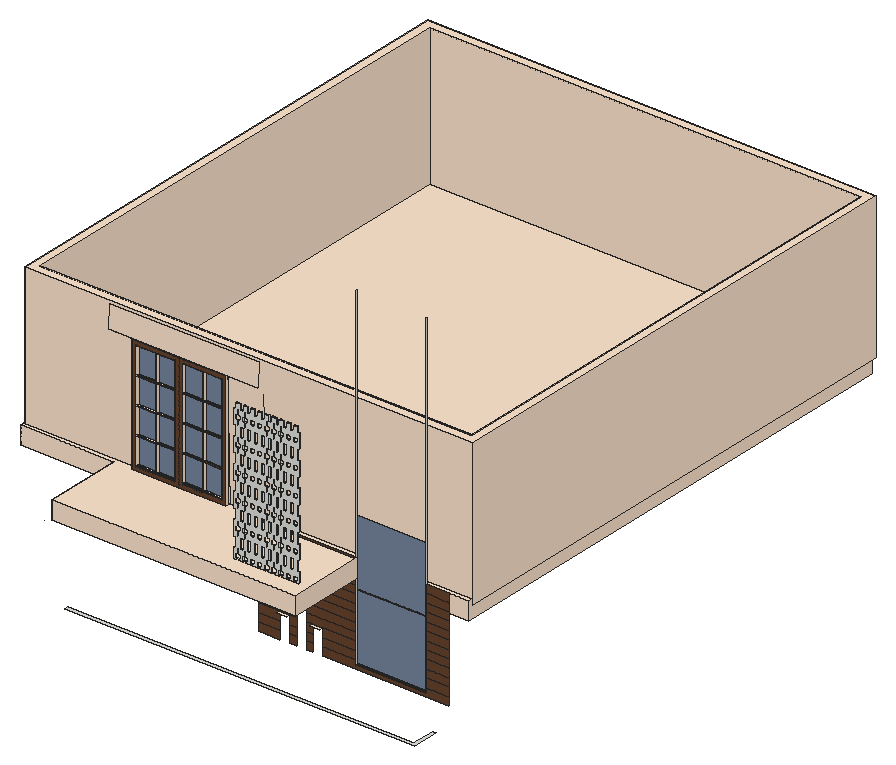
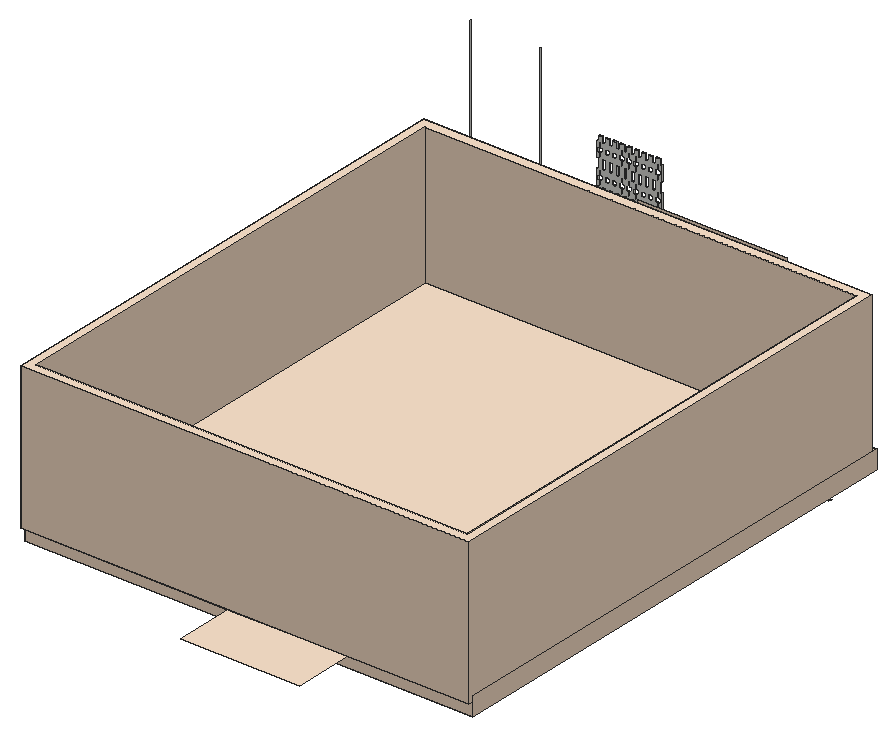
# SketchUp Ruby script. Lengths in inches.
U = 1.inch
M = Sketchup.active_model
def pt(a) = Geom::Point3d.new(a.map { |v| v * U })
def face(e, loops, mat)
  f = e.add_face(loops[0].map { |a| pt(a) })
  loops[1..].each { |l| e.add_face(l.map { |a| pt(a) }).erase! }
  f.material = f.back_material = mat if mat
  f
end
# faces: each face lists its corners as indices into pts; further lists are holes
def faces(e, pts, list, mat = nil) = list.each { |f| face(e, (f[0].is_a?(Array) ? f : [f]).map { |l| l.map { |i| pts[i] } }, mat) }
# xy, xz, yz: faces in a plane at the given z, y or x. An outline is a flat list of corners, or four numbers for a rectangle; further outlines are holes
def ring(l) = l.size == 4 ? [[l[0], l[1]], [l[2], l[1]], [l[2], l[3]], [l[0], l[3]]] : l.each_slice(2).to_a
def flat(e, list, mat, &to3) = list.each { |f| face(e, (f[0].is_a?(Array) ? f : [f]).map { |l| ring(l).map { |u, v| to3.(u, v) } }, mat) }
def xy(e, z, list, mat = nil) = flat(e, list, mat) { |x, y| [x, y, z] }
def xz(e, y, list, mat = nil) = flat(e, list, mat) { |x, z| [x, y, z] }
def yz(e, x, list, mat = nil) = flat(e, list, mat) { |y, z| [x, y, z] }
def lines(e, pts, list) = list.each { |a, b| e.add_line(pt(pts[a]), pt(pts[b])) }
# prism: a flat outline (further loops are holes) pulled along v
def prism(e, loops, v, mat = nil)
  f = face(e, loops, mat); d = Geom::Vector3d.new(v.map { |x| x * U })
  f.pushpull(f.normal.samedirection?(d) ? d.length : -d.length)
end
def box(e, o, s, mat = nil) = prism(e, [[o, [o[0] + s[0], o[1], o[2]], [o[0] + s[0], o[1] + s[1], o[2]], [o[0], o[1] + s[1], o[2]]]], [0, 0, s[2]], mat)
def at(x, y, z, deg = 0) = Geom::Transformation.translation(pt([x, y, z])) * Geom::Transformation.rotation(ORIGIN, Z_AXIS, deg.degrees)
def axes(o, x, y, z) = Geom::Transformation.new([*x, 0, *y, 0, *z, 0, *pt(o).to_a, 1])
def part(name) = M.definitions.add(name)
# library, detail: a bought-in or finely detailed component or shape, given as its bounding box
def library(name, o, s) = part(name).tap { |d| box(d.entities, o, s) }
def detail(e, o, s) = box(e.add_group.entities, o, s)
def put(e, d, t, mat = nil) = e.add_instance(d, t).tap { |i| i.material = mat if mat }
def group(e, t, mat = nil) = e.add_group.tap { |g| g.transformation = t; g.material = mat if mat }.entities
root = M.entities
M.materials.add("C01_Vanilla_Cream").color = [255, 230, 206]
M.materials.add("Glass_Mirror_01").color = [119, 135, 160]
M.materials.add("Wood_Veneer_15_1K").color = [103, 69, 45]
xy(root,193.67,[[105.48,138.27,465.23,138.27,465.23,165.41,462.4,165.41,462.4,141.07,105.48,141.07]])
xy(root,203.87,[[357,198,429,199.5]])
xy(root,225.8,[[278.18,194.51,288.54,198],[312.12,194.51,322.48,198]],"C01_Vanilla_Cream")
xy(root,243.16,[[296.18,194.51,306.54,198]],"C01_Vanilla_Cream")
xy(root,292.23,[[282.27,137.21,285.76,138.74],[289.68,137.21,293.17,138.74],[297.09,137.21,300.58,138.74],[304.5,137.21,307.99,138.74],[311.91,137.21,315.4,138.74],
  [319.32,137.21,322.81,138.74],[326.73,137.21,330.22,138.74],[334.14,137.21,337.63,138.74],[341.55,137.21,345.04,138.74]])
xz(root,137.21,[[[282.27,292.23,285.76,292.23,285.76,297.49,289.68,297.49,289.68,292.23,293.17,292.23,293.17,297.49,297.09,297.49,297.09,292.23,300.58,292.23,300.58,297.49,304.5,297.49,304.5,292.23,307.99,292.23,307.99,297.49,311.91,297.49,311.91,292.23,315.4,292.23,315.4,297.49,319.32,297.49,319.32,292.23,322.81,292.23,322.81,297.49,326.73,297.49,326.73,292.23,330.22,292.23,330.22,297.49,334.14,297.49,334.14,292.23,337.63,292.23,337.63,297.49,341.55,297.49,341.55,292.23,345.04,292.23,345.04,297.49,347,297.49,347,312.59,345.04,312.59,345.04,323.12,347,323.12,347,338.22,345.04,338.22,345.04,348.75,347,348.75,347,363.84,345.04,363.84,345.04,374.38,347,374.38,347,389.47,345.04,389.47,345.04,400.01,347,400.01,347,415.1,345.04,415.1,345.04,425.64,347,425.64,347,440.73,345.04,440.73,345.04,446,341.55,446,341.55,440.73,337.63,440.73,337.63,446,334.14,446,334.14,440.73,330.22,440.73,330.22,446,326.73,446,326.73,440.73,322.81,440.73,322.81,446,319.32,446,319.32,440.73,315.4,440.73,315.4,446,311.91,446,311.91,440.73,307.99,440.73,307.99,446,304.5,446,304.5,440.73,300.58,440.73,300.58,446,297.09,446,297.09,440.73,293.17,440.73,293.17,446,289.68,446,289.68,440.73,285.76,440.73,285.76,446,282.27,446,282.27,440.73,280.31,440.73,280.31,425.64,282.27,425.64,282.27,415.1,280.31,415.1,280.31,400.01,282.27,400.01,282.27,389.47,280.31,389.47,280.31,374.38,282.27,374.38,282.27,363.84,280.31,363.84,280.31,348.75,282.27,348.75,282.27,338.22,280.31,338.22,280.31,323.12,282.27,323.12,282.27,312.59,280.31,312.59,280.31,297.49,282.27,297.49],[312.78,297.09,312.78,302.36,310.82,302.36,310.82,307.72,312.78,307.72,312.78,312.99,314.53,312.99,314.53,307.72,316.49,307.72,316.49,302.36,314.53,302.36,314.53,297.09],[305.37,297.09,305.37,302.36,303.41,302.36,303.41,307.72,305.37,307.72,305.37,312.99,307.12,312.99,307.12,307.72,309.08,307.72,309.08,302.36,307.12,302.36,307.12,297.09],[312.78,399.61,312.78,404.88,310.82,404.88,310.82,410.24,312.78,410.24,312.78,415.5,314.53,415.5,314.53,410.24,316.49,410.24,316.49,404.88,314.53,404.88,314.53,399.61],[312.78,373.98,312.78,379.25,310.82,379.25,310.82,384.61,312.78,384.61,312.78,389.875,314.53,389.875,314.53,384.61,316.49,384.61,316.49,379.25,314.53,379.25,314.53,373.98],[312.78,425.24,312.78,430.51,310.82,430.51,310.82,435.86,312.78,435.86,312.78,441.13,314.53,441.13,314.53,435.86,316.49,435.86,316.49,430.51,314.53,430.51,314.53,425.24],[312.78,322.72,312.78,327.99,310.82,327.99,310.82,333.35,312.78,333.35,312.78,338.62,314.53,338.62,314.53,333.35,316.49,333.35,316.49,327.99,314.53,327.99,314.53,322.72],[305.37,399.61,305.37,404.88,303.41,404.88,303.41,410.24,305.37,410.24,305.37,415.5,307.12,415.5,307.12,410.24,309.08,410.24,309.08,404.88,307.12,404.88,307.12,399.61],[305.37,373.98,305.37,379.25,303.41,379.25,303.41,384.61,305.37,384.61,305.37,389.875,307.12,389.875,307.12,384.61,309.08,384.61,309.08,379.25,307.12,379.25,307.12,373.98],[305.37,425.24,305.37,430.51,303.41,430.51,303.41,435.86,305.37,435.86,305.37,441.13,307.12,441.13,307.12,435.86,309.08,435.86,309.08,430.51,307.12,430.51,307.12,425.24],[305.37,322.72,305.37,327.99,303.41,327.99,303.41,333.35,305.37,333.35,305.37,338.62,307.12,338.62,307.12,333.35,309.08,333.35,309.08,327.99,307.12,327.99,307.12,322.72],[312.78,348.35,312.78,353.62,310.82,353.62,310.82,358.98,312.78,358.98,312.78,364.24,314.53,364.24,314.53,358.98,316.49,358.98,316.49,353.62,314.53,353.62,314.53,348.35],[305.37,348.35,305.37,353.62,303.41,353.62,303.41,358.98,305.37,358.98,305.37,364.24,307.12,364.24,307.12,358.98,309.08,358.98,309.08,353.62,307.12,353.62,307.12,348.35],[342.42,297.09,342.42,302.36,340.46,302.36,340.46,307.72,342.42,307.72,342.42,312.99,344.17,312.99,344.17,307.72,346.13,307.72,346.13,302.36,344.17,302.36,344.17,297.09],[342.42,399.61,342.42,404.88,340.46,404.88,340.46,410.24,342.42,410.24,342.42,415.5,344.17,415.5,344.17,410.24,346.13,410.24,346.13,404.88,344.17,404.88,344.17,399.61],[342.42,425.24,342.42,430.51,340.46,430.51,340.46,435.86,342.42,435.86,342.42,441.13,344.17,441.13,344.17,435.86,346.13,435.86,346.13,430.51,344.17,430.51,344.17,425.24],[342.42,373.98,342.42,379.25,340.46,379.25,340.46,384.61,342.42,384.61,342.42,389.875,344.17,389.875,344.17,384.61,346.13,384.61,346.13,379.25,344.17,379.25,344.17,373.98],[342.42,322.72,342.42,327.99,340.46,327.99,340.46,333.35,342.42,333.35,342.42,338.62,344.17,338.62,344.17,333.35,346.13,333.35,346.13,327.99,344.17,327.99,344.17,322.72],[290.55,297.09,290.55,302.36,288.59,302.36,288.59,307.72,290.55,307.72,290.55,312.99,292.3,312.99,292.3,307.72,294.26,307.72,294.26,302.36,292.3,302.36,292.3,297.09],[290.55,399.61,290.55,404.88,288.59,404.88,288.59,410.24,290.55,410.24,290.55,415.5,292.3,415.5,292.3,410.24,294.26,410.24,294.26,404.88,292.3,404.88,292.3,399.61],[290.55,373.98,290.55,379.25,288.59,379.25,288.59,384.61,290.55,384.61,290.55,389.875,292.3,389.875,292.3,384.61,294.26,384.61,294.26,379.25,292.3,379.25,292.3,373.98],[290.55,425.24,290.55,430.51,288.59,430.51,288.59,435.86,290.55,435.86,290.55,441.13,292.3,441.13,292.3,435.86,294.26,435.86,294.26,430.51,292.3,430.51,292.3,425.24],[342.42,348.35,342.42,353.62,340.46,353.62,340.46,358.98,342.42,358.98,342.42,364.24,344.17,364.24,344.17,358.98,346.13,358.98,346.13,353.62,344.17,353.62,344.17,348.35],[290.55,322.72,290.55,327.99,288.59,327.99,288.59,333.35,290.55,333.35,290.55,338.62,292.3,338.62,292.3,333.35,294.26,333.35,294.26,327.99,292.3,327.99,292.3,322.72],[290.55,348.35,290.55,353.62,288.59,353.62,288.59,358.98,290.55,358.98,290.55,364.24,292.3,364.24,292.3,358.98,294.26,358.98,294.26,353.62,292.3,353.62,292.3,348.35],[335.01,297.09,335.01,302.36,333.05,302.36,333.05,307.72,335.01,307.72,335.01,312.99,336.76,312.99,336.76,307.72,338.72,307.72,338.72,302.36,336.76,302.36,336.76,297.09],[335.01,425.24,335.01,430.51,333.05,430.51,333.05,435.86,335.01,435.86,335.01,441.13,336.76,441.13,336.76,435.86,338.72,435.86,338.72,430.51,336.76,430.51,336.76,425.24],[327.6,297.09,327.6,302.36,325.64,302.36,325.64,307.72,327.6,307.72,327.6,312.99,329.35,312.99,329.35,307.72,331.31,307.72,331.31,302.36,329.35,302.36,329.35,297.09],[335.01,399.61,335.01,404.88,333.05,404.88,333.05,410.24,335.01,410.24,335.01,415.5,336.76,415.5,336.76,410.24,338.72,410.24,338.72,404.88,336.76,404.88,336.76,399.61],[335.01,373.98,335.01,379.25,333.05,379.25,333.05,384.61,335.01,384.61,335.01,389.875,336.76,389.875,336.76,384.61,338.72,384.61,338.72,379.25,336.76,379.25,336.76,373.98],[335.01,322.72,335.01,327.99,333.05,327.99,333.05,333.35,335.01,333.35,335.01,338.62,336.76,338.62,336.76,333.35,338.72,333.35,338.72,327.99,336.76,327.99,336.76,322.72],[327.6,373.98,327.6,379.25,325.64,379.25,325.64,384.61,327.6,384.61,327.6,389.875,329.35,389.875,329.35,384.61,331.31,384.61,331.31,379.25,329.35,379.25,329.35,373.98],[327.6,399.61,327.6,404.88,325.64,404.88,325.64,410.24,327.6,410.24,327.6,415.5,329.35,415.5,329.35,410.24,331.31,410.24,331.31,404.88,329.35,404.88,329.35,399.61],[327.6,425.24,327.6,430.51,325.64,430.51,325.64,435.86,327.6,435.86,327.6,441.13,329.35,441.13,329.35,435.86,331.31,435.86,331.31,430.51,329.35,430.51,329.35,425.24],[327.6,322.72,327.6,327.99,325.64,327.99,325.64,333.35,327.6,333.35,327.6,338.62,329.35,338.62,329.35,333.35,331.31,333.35,331.31,327.99,329.35,327.99,329.35,322.72],[283.14,297.09,283.14,302.36,281.18,302.36,281.18,307.72,283.14,307.72,283.14,312.99,284.89,312.99,284.89,307.72,286.85,307.72,286.85,302.36,284.89,302.36,284.89,297.09],[335.01,348.35,335.01,353.62,333.05,353.62,333.05,358.98,335.01,358.98,335.01,364.24,336.76,364.24,336.76,358.98,338.72,358.98,338.72,353.62,336.76,353.62,336.76,348.35],[283.14,399.61,283.14,404.88,281.18,404.88,281.18,410.24,283.14,410.24,283.14,415.5,284.89,415.5,284.89,410.24,286.85,410.24,286.85,404.88,284.89,404.88,284.89,399.61],[320.1875,297.09,320.1875,302.36,318.23,302.36,318.23,307.72,320.1875,307.72,320.1875,312.99,321.94,312.99,321.94,307.72,323.9,307.72,323.9,302.36,321.94,302.36,321.94,297.09],[283.14,373.98,283.14,379.25,281.18,379.25,281.18,384.61,283.14,384.61,283.14,389.875,284.89,389.875,284.89,384.61,286.85,384.61,286.85,379.25,284.89,379.25,284.89,373.98],[283.14,425.24,283.14,430.51,281.18,430.51,281.18,435.86,283.14,435.86,283.14,441.13,284.89,441.13,284.89,435.86,286.85,435.86,286.85,430.51,284.89,430.51,284.89,425.24],[327.6,348.35,327.6,353.62,325.64,353.62,325.64,358.98,327.6,358.98,327.6,364.24,329.35,364.24,329.35,358.98,331.31,358.98,331.31,353.62,329.35,353.62,329.35,348.35],[283.14,322.72,283.14,327.99,281.18,327.99,281.18,333.35,283.14,333.35,283.14,338.62,284.89,338.62,284.89,333.35,286.85,333.35,286.85,327.99,284.89,327.99,284.89,322.72],[320.1875,399.61,320.1875,404.88,318.23,404.88,318.23,410.24,320.1875,410.24,320.1875,415.5,321.94,415.5,321.94,410.24,323.9,410.24,323.9,404.88,321.94,404.88,321.94,399.61],[320.1875,425.24,320.1875,430.51,318.23,430.51,318.23,435.86,320.1875,435.86,320.1875,441.13,321.94,441.13,321.94,435.86,323.9,435.86,323.9,430.51,321.94,430.51,321.94,425.24],[320.1875,373.98,320.1875,379.25,318.23,379.25,318.23,384.61,320.1875,384.61,320.1875,389.875,321.94,389.875,321.94,384.61,323.9,384.61,323.9,379.25,321.94,379.25,321.94,373.98],[320.1875,322.72,320.1875,327.99,318.23,327.99,318.23,333.35,320.1875,333.35,320.1875,338.62,321.94,338.62,321.94,333.35,323.9,333.35,323.9,327.99,321.94,327.99,321.94,322.72],[283.14,348.35,283.14,353.62,281.18,353.62,281.18,358.98,283.14,358.98,283.14,364.24,284.89,364.24,284.89,358.98,286.85,358.98,286.85,353.62,284.89,353.62,284.89,348.35],[297.96,297.09,297.96,302.36,296,302.36,296,307.72,297.96,307.72,297.96,312.99,299.71,312.99,299.71,307.72,301.67,307.72,301.67,302.36,299.71,302.36,299.71,297.09],[320.1875,348.35,320.1875,353.62,318.23,353.62,318.23,358.98,320.1875,358.98,320.1875,364.24,321.94,364.24,321.94,358.98,323.9,358.98,323.9,353.62,321.94,353.62,321.94,348.35],[297.96,399.61,297.96,404.88,296,404.88,296,410.24,297.96,410.24,297.96,415.5,299.71,415.5,299.71,410.24,301.67,410.24,301.67,404.88,299.71,404.88,299.71,399.61],[297.96,425.24,297.96,430.51,296,430.51,296,435.86,297.96,435.86,297.96,441.13,299.71,441.13,299.71,435.86,301.67,435.86,301.67,430.51,299.71,430.51,299.71,425.24],[297.96,373.98,297.96,379.25,296,379.25,296,384.61,297.96,384.61,297.96,389.875,299.71,389.875,299.71,384.61,301.67,384.61,301.67,379.25,299.71,379.25,299.71,373.98],[297.96,322.72,297.96,327.99,296,327.99,296,333.35,297.96,333.35,297.96,338.62,299.71,338.62,299.71,333.35,301.67,333.35,301.67,327.99,299.71,327.99,299.71,322.72],[297.96,348.35,297.96,353.62,296,353.62,296,358.98,297.96,358.98,297.96,364.24,299.71,364.24,299.71,358.98,301.67,358.98,301.67,353.62,299.71,353.62,299.71,348.35],[330.22,363.84,334.14,374.38],[307.99,363.84,311.91,374.38],[330.22,338.22,334.14,348.75],[330.22,389.47,334.14,400.01],[307.99,338.22,311.91,348.75],[307.99,389.47,311.91,400.01],[330.22,415.1,334.14,425.64],[307.99,415.1,311.91,425.64],[330.22,312.59,334.14,323.12],[307.99,312.59,311.91,323.12],[300.58,363.84,304.5,374.38],[300.58,338.22,304.5,348.75],[300.58,389.47,304.5,400.01],[300.58,415.1,304.5,425.64],[300.58,312.59,304.5,323.12],[315.4,363.84,319.32,374.38],[315.4,389.47,319.32,400.01],[285.76,363.84,289.68,374.38],[315.4,415.1,319.32,425.64],[285.76,338.22,289.68,348.75],[315.4,338.22,319.32,348.75],[285.76,389.47,289.68,400.01],[285.76,415.1,289.68,425.64],[315.4,312.59,319.32,323.12],[293.17,363.84,297.09,374.38],[322.81,363.84,326.73,374.38],[322.81,338.22,326.73,348.75],[285.76,312.59,289.68,323.12],[293.17,389.47,297.09,400.01],[322.81,389.47,326.73,400.01],[322.81,415.1,326.73,425.64],[293.17,415.1,297.09,425.64],[293.17,338.22,297.09,348.75],[293.17,312.59,297.09,323.12],[322.81,312.59,326.73,323.12],[337.63,363.84,341.55,374.38],[337.63,389.47,341.55,400.01],[337.63,415.1,341.55,425.64],[337.63,338.22,341.55,348.75],[337.63,312.59,341.55,323.12]]])
xz(root,138.74,[[[282.27,292.23,282.27,297.49,280.31,297.49,280.31,312.59,282.27,312.59,282.27,323.12,280.31,323.12,280.31,338.22,282.27,338.22,282.27,348.75,280.31,348.75,280.31,363.84,282.27,363.84,282.27,374.38,280.31,374.38,280.31,389.47,282.27,389.47,282.27,400.01,280.31,400.01,280.31,415.1,282.27,415.1,282.27,425.64,280.31,425.64,280.31,440.73,282.27,440.73,282.27,446,285.76,446,285.76,440.73,289.68,440.73,289.68,446,293.17,446,293.17,440.73,297.09,440.73,297.09,446,300.58,446,300.58,440.73,304.5,440.73,304.5,446,307.99,446,307.99,440.73,311.91,440.73,311.91,446,315.4,446,315.4,440.73,319.32,440.73,319.32,446,322.81,446,322.81,440.73,326.73,440.73,326.73,446,330.22,446,330.22,440.73,334.14,440.73,334.14,446,337.63,446,337.63,440.73,341.55,440.73,341.55,446,345.04,446,345.04,440.73,347,440.73,347,425.64,345.04,425.64,345.04,415.1,347,415.1,347,400.01,345.04,400.01,345.04,389.47,347,389.47,347,374.38,345.04,374.38,345.04,363.84,347,363.84,347,348.75,345.04,348.75,345.04,338.22,347,338.22,347,323.12,345.04,323.12,345.04,312.59,347,312.59,347,297.49,345.04,297.49,345.04,292.23,341.55,292.23,341.55,297.49,337.63,297.49,337.63,292.23,334.14,292.23,334.14,297.49,330.22,297.49,330.22,292.23,326.73,292.23,326.73,297.49,322.81,297.49,322.81,292.23,319.32,292.23,319.32,297.49,315.4,297.49,315.4,292.23,311.91,292.23,311.91,297.49,307.99,297.49,307.99,292.23,304.5,292.23,304.5,297.49,300.58,297.49,300.58,292.23,297.09,292.23,297.09,297.49,293.17,297.49,293.17,292.23,289.68,292.23,289.68,297.49,285.76,297.49,285.76,292.23],[312.78,297.09,314.53,297.09,314.53,302.36,316.49,302.36,316.49,307.72,314.53,307.72,314.53,312.99,312.78,312.99,312.78,307.72,310.82,307.72,310.82,302.36,312.78,302.36],[305.37,297.09,307.12,297.09,307.12,302.36,309.08,302.36,309.08,307.72,307.12,307.72,307.12,312.99,305.37,312.99,305.37,307.72,303.41,307.72,303.41,302.36,305.37,302.36],[312.78,399.61,314.53,399.61,314.53,404.88,316.49,404.88,316.49,410.24,314.53,410.24,314.53,415.5,312.78,415.5,312.78,410.24,310.82,410.24,310.82,404.88,312.78,404.88],[312.78,373.98,314.53,373.98,314.53,379.25,316.49,379.25,316.49,384.61,314.53,384.61,314.53,389.875,312.78,389.875,312.78,384.61,310.82,384.61,310.82,379.25,312.78,379.25],[312.78,425.24,314.53,425.24,314.53,430.51,316.49,430.51,316.49,435.86,314.53,435.86,314.53,441.13,312.78,441.13,312.78,435.86,310.82,435.86,310.82,430.51,312.78,430.51],[305.37,399.61,307.12,399.61,307.12,404.88,309.08,404.88,309.08,410.24,307.12,410.24,307.12,415.5,305.37,415.5,305.37,410.24,303.41,410.24,303.41,404.88,305.37,404.88],[312.78,322.72,314.53,322.72,314.53,327.99,316.49,327.99,316.49,333.35,314.53,333.35,314.53,338.62,312.78,338.62,312.78,333.35,310.82,333.35,310.82,327.99,312.78,327.99],[305.37,373.98,307.12,373.98,307.12,379.25,309.08,379.25,309.08,384.61,307.12,384.61,307.12,389.875,305.37,389.875,305.37,384.61,303.41,384.61,303.41,379.25,305.37,379.25],[305.37,425.24,307.12,425.24,307.12,430.51,309.08,430.51,309.08,435.86,307.12,435.86,307.12,441.13,305.37,441.13,305.37,435.86,303.41,435.86,303.41,430.51,305.37,430.51],[305.37,322.72,307.12,322.72,307.12,327.99,309.08,327.99,309.08,333.35,307.12,333.35,307.12,338.62,305.37,338.62,305.37,333.35,303.41,333.35,303.41,327.99,305.37,327.99],[312.78,348.35,314.53,348.35,314.53,353.62,316.49,353.62,316.49,358.98,314.53,358.98,314.53,364.24,312.78,364.24,312.78,358.98,310.82,358.98,310.82,353.62,312.78,353.62],[305.37,348.35,307.12,348.35,307.12,353.62,309.08,353.62,309.08,358.98,307.12,358.98,307.12,364.24,305.37,364.24,305.37,358.98,303.41,358.98,303.41,353.62,305.37,353.62],[342.42,297.09,344.17,297.09,344.17,302.36,346.13,302.36,346.13,307.72,344.17,307.72,344.17,312.99,342.42,312.99,342.42,307.72,340.46,307.72,340.46,302.36,342.42,302.36],[342.42,399.61,344.17,399.61,344.17,404.88,346.13,404.88,346.13,410.24,344.17,410.24,344.17,415.5,342.42,415.5,342.42,410.24,340.46,410.24,340.46,404.88,342.42,404.88],[342.42,425.24,344.17,425.24,344.17,430.51,346.13,430.51,346.13,435.86,344.17,435.86,344.17,441.13,342.42,441.13,342.42,435.86,340.46,435.86,340.46,430.51,342.42,430.51],[342.42,373.98,344.17,373.98,344.17,379.25,346.13,379.25,346.13,384.61,344.17,384.61,344.17,389.875,342.42,389.875,342.42,384.61,340.46,384.61,340.46,379.25,342.42,379.25],[342.42,322.72,344.17,322.72,344.17,327.99,346.13,327.99,346.13,333.35,344.17,333.35,344.17,338.62,342.42,338.62,342.42,333.35,340.46,333.35,340.46,327.99,342.42,327.99],[290.55,297.09,292.3,297.09,292.3,302.36,294.26,302.36,294.26,307.72,292.3,307.72,292.3,312.99,290.55,312.99,290.55,307.72,288.59,307.72,288.59,302.36,290.55,302.36],[290.55,399.61,292.3,399.61,292.3,404.88,294.26,404.88,294.26,410.24,292.3,410.24,292.3,415.5,290.55,415.5,290.55,410.24,288.59,410.24,288.59,404.88,290.55,404.88],[290.55,373.98,292.3,373.98,292.3,379.25,294.26,379.25,294.26,384.61,292.3,384.61,292.3,389.875,290.55,389.875,290.55,384.61,288.59,384.61,288.59,379.25,290.55,379.25],[290.55,425.24,292.3,425.24,292.3,430.51,294.26,430.51,294.26,435.86,292.3,435.86,292.3,441.13,290.55,441.13,290.55,435.86,288.59,435.86,288.59,430.51,290.55,430.51],[342.42,348.35,344.17,348.35,344.17,353.62,346.13,353.62,346.13,358.98,344.17,358.98,344.17,364.24,342.42,364.24,342.42,358.98,340.46,358.98,340.46,353.62,342.42,353.62],[290.55,322.72,292.3,322.72,292.3,327.99,294.26,327.99,294.26,333.35,292.3,333.35,292.3,338.62,290.55,338.62,290.55,333.35,288.59,333.35,288.59,327.99,290.55,327.99],[290.55,348.35,292.3,348.35,292.3,353.62,294.26,353.62,294.26,358.98,292.3,358.98,292.3,364.24,290.55,364.24,290.55,358.98,288.59,358.98,288.59,353.62,290.55,353.62],[335.01,297.09,336.76,297.09,336.76,302.36,338.72,302.36,338.72,307.72,336.76,307.72,336.76,312.99,335.01,312.99,335.01,307.72,333.05,307.72,333.05,302.36,335.01,302.36],[327.6,297.09,329.35,297.09,329.35,302.36,331.31,302.36,331.31,307.72,329.35,307.72,329.35,312.99,327.6,312.99,327.6,307.72,325.64,307.72,325.64,302.36,327.6,302.36],[335.01,425.24,336.76,425.24,336.76,430.51,338.72,430.51,338.72,435.86,336.76,435.86,336.76,441.13,335.01,441.13,335.01,435.86,333.05,435.86,333.05,430.51,335.01,430.51],[335.01,399.61,336.76,399.61,336.76,404.88,338.72,404.88,338.72,410.24,336.76,410.24,336.76,415.5,335.01,415.5,335.01,410.24,333.05,410.24,333.05,404.88,335.01,404.88],[335.01,373.98,336.76,373.98,336.76,379.25,338.72,379.25,338.72,384.61,336.76,384.61,336.76,389.875,335.01,389.875,335.01,384.61,333.05,384.61,333.05,379.25,335.01,379.25],[335.01,322.72,336.76,322.72,336.76,327.99,338.72,327.99,338.72,333.35,336.76,333.35,336.76,338.62,335.01,338.62,335.01,333.35,333.05,333.35,333.05,327.99,335.01,327.99],[327.6,373.98,329.35,373.98,329.35,379.25,331.31,379.25,331.31,384.61,329.35,384.61,329.35,389.875,327.6,389.875,327.6,384.61,325.64,384.61,325.64,379.25,327.6,379.25],[327.6,425.24,329.35,425.24,329.35,430.51,331.31,430.51,331.31,435.86,329.35,435.86,329.35,441.13,327.6,441.13,327.6,435.86,325.64,435.86,325.64,430.51,327.6,430.51],[327.6,399.61,329.35,399.61,329.35,404.88,331.31,404.88,331.31,410.24,329.35,410.24,329.35,415.5,327.6,415.5,327.6,410.24,325.64,410.24,325.64,404.88,327.6,404.88],[327.6,322.72,329.35,322.72,329.35,327.99,331.31,327.99,331.31,333.35,329.35,333.35,329.35,338.62,327.6,338.62,327.6,333.35,325.64,333.35,325.64,327.99,327.6,327.99],[283.14,297.09,284.89,297.09,284.89,302.36,286.85,302.36,286.85,307.72,284.89,307.72,284.89,312.99,283.14,312.99,283.14,307.72,281.18,307.72,281.18,302.36,283.14,302.36],[335.01,348.35,336.76,348.35,336.76,353.62,338.72,353.62,338.72,358.98,336.76,358.98,336.76,364.24,335.01,364.24,335.01,358.98,333.05,358.98,333.05,353.62,335.01,353.62],[283.14,399.61,284.89,399.61,284.89,404.88,286.85,404.88,286.85,410.24,284.89,410.24,284.89,415.5,283.14,415.5,283.14,410.24,281.18,410.24,281.18,404.88,283.14,404.88],[320.1875,297.09,321.94,297.09,321.94,302.36,323.9,302.36,323.9,307.72,321.94,307.72,321.94,312.99,320.1875,312.99,320.1875,307.72,318.23,307.72,318.23,302.36,320.1875,302.36],[283.14,373.98,284.89,373.98,284.89,379.25,286.85,379.25,286.85,384.61,284.89,384.61,284.89,389.875,283.14,389.875,283.14,384.61,281.18,384.61,281.18,379.25,283.14,379.25],[283.14,425.24,284.89,425.24,284.89,430.51,286.85,430.51,286.85,435.86,284.89,435.86,284.89,441.13,283.14,441.13,283.14,435.86,281.18,435.86,281.18,430.51,283.14,430.51],[327.6,348.35,329.35,348.35,329.35,353.62,331.31,353.62,331.31,358.98,329.35,358.98,329.35,364.24,327.6,364.24,327.6,358.98,325.64,358.98,325.64,353.62,327.6,353.62],[283.14,322.72,284.89,322.72,284.89,327.99,286.85,327.99,286.85,333.35,284.89,333.35,284.89,338.62,283.14,338.62,283.14,333.35,281.18,333.35,281.18,327.99,283.14,327.99],[320.1875,399.61,321.94,399.61,321.94,404.88,323.9,404.88,323.9,410.24,321.94,410.24,321.94,415.5,320.1875,415.5,320.1875,410.24,318.23,410.24,318.23,404.88,320.1875,404.88],[320.1875,373.98,321.94,373.98,321.94,379.25,323.9,379.25,323.9,384.61,321.94,384.61,321.94,389.875,320.1875,389.875,320.1875,384.61,318.23,384.61,318.23,379.25,320.1875,379.25],[320.1875,425.24,321.94,425.24,321.94,430.51,323.9,430.51,323.9,435.86,321.94,435.86,321.94,441.13,320.1875,441.13,320.1875,435.86,318.23,435.86,318.23,430.51,320.1875,430.51],[320.1875,322.72,321.94,322.72,321.94,327.99,323.9,327.99,323.9,333.35,321.94,333.35,321.94,338.62,320.1875,338.62,320.1875,333.35,318.23,333.35,318.23,327.99,320.1875,327.99],[283.14,348.35,284.89,348.35,284.89,353.62,286.85,353.62,286.85,358.98,284.89,358.98,284.89,364.24,283.14,364.24,283.14,358.98,281.18,358.98,281.18,353.62,283.14,353.62],[297.96,297.09,299.71,297.09,299.71,302.36,301.67,302.36,301.67,307.72,299.71,307.72,299.71,312.99,297.96,312.99,297.96,307.72,296,307.72,296,302.36,297.96,302.36],[320.1875,348.35,321.94,348.35,321.94,353.62,323.9,353.62,323.9,358.98,321.94,358.98,321.94,364.24,320.1875,364.24,320.1875,358.98,318.23,358.98,318.23,353.62,320.1875,353.62],[297.96,399.61,299.71,399.61,299.71,404.88,301.67,404.88,301.67,410.24,299.71,410.24,299.71,415.5,297.96,415.5,297.96,410.24,296,410.24,296,404.88,297.96,404.88],[297.96,373.98,299.71,373.98,299.71,379.25,301.67,379.25,301.67,384.61,299.71,384.61,299.71,389.875,297.96,389.875,297.96,384.61,296,384.61,296,379.25,297.96,379.25],[297.96,425.24,299.71,425.24,299.71,430.51,301.67,430.51,301.67,435.86,299.71,435.86,299.71,441.13,297.96,441.13,297.96,435.86,296,435.86,296,430.51,297.96,430.51],[297.96,322.72,299.71,322.72,299.71,327.99,301.67,327.99,301.67,333.35,299.71,333.35,299.71,338.62,297.96,338.62,297.96,333.35,296,333.35,296,327.99,297.96,327.99],[297.96,348.35,299.71,348.35,299.71,353.62,301.67,353.62,301.67,358.98,299.71,358.98,299.71,364.24,297.96,364.24,297.96,358.98,296,358.98,296,353.62,297.96,353.62],[330.22,363.84,334.14,374.38],[307.99,363.84,311.91,374.38],[330.22,338.22,334.14,348.75],[330.22,389.47,334.14,400.01],[307.99,338.22,311.91,348.75],[307.99,389.47,311.91,400.01],[330.22,415.1,334.14,425.64],[307.99,415.1,311.91,425.64],[330.22,312.59,334.14,323.12],[307.99,312.59,311.91,323.12],[300.58,363.84,304.5,374.38],[300.58,338.22,304.5,348.75],[300.58,389.47,304.5,400.01],[300.58,415.1,304.5,425.64],[300.58,312.59,304.5,323.12],[315.4,363.84,319.32,374.38],[315.4,389.47,319.32,400.01],[285.76,363.84,289.68,374.38],[315.4,415.1,319.32,425.64],[285.76,338.22,289.68,348.75],[315.4,338.22,319.32,348.75],[285.76,389.47,289.68,400.01],[285.76,415.1,289.68,425.64],[315.4,312.59,319.32,323.12],[293.17,363.84,297.09,374.38],[322.81,363.84,326.73,374.38],[322.81,338.22,326.73,348.75],[285.76,312.59,289.68,323.12],[293.17,389.47,297.09,400.01],[322.81,389.47,326.73,400.01],[322.81,415.1,326.73,425.64],[293.17,415.1,297.09,425.64],[293.17,338.22,297.09,348.75],[293.17,312.59,297.09,323.12],[322.81,312.59,326.73,323.12],[337.63,363.84,341.55,374.38],[337.63,389.47,341.55,400.01],[337.63,415.1,341.55,425.64],[337.63,338.22,341.55,348.75],[337.63,312.59,341.55,323.12]]])
xz(root,198,[[256.9,199.76,278.18,208.44],[288.54,199.76,296.18,208.44],[306.54,199.76,312.12,208.44],[322.48,199.76,453,199.76,453,208.44,429,208.44,429,203.87,357,203.87,357,208.44,322.48,208.44],[256.9,208.44,278.18,217.12],
  [288.54,208.44,296.18,217.12],[306.54,208.44,312.12,217.12],[322.48,208.44,357,217.12],[429,208.44,453,217.12],[256.9,217.12,278.18,225.8],
  [288.54,217.12,296.18,225.8],[306.54,217.12,312.12,225.8],[322.48,217.12,357,225.8],[429,217.12,453,225.8],[256.9,225.8,296.18,234.48],
  [306.54,225.8,357,234.48],[429,225.8,453,234.48],[256.9,234.48,296.18,243.16],[306.54,234.48,357,243.16],[429,234.48,453,243.16],
  [256.9,243.16,357,251.84],[429,243.16,453,251.84],[256.9,251.84,357,260.52],[429,251.84,453,260.52],[256.9,260.52,357,269.2],
  [429,260.52,453,269.2],[256.9,269.2,357,277.88],[429,269.2,453,277.88],[256.9,277.88,357,286.56],[429,277.88,453,286.56],
  [256.9,286.56,357,295.24],[429,286.56,453,295.24],[256.9,295.24,357,303.92],[429,295.24,453,303.92]],"Wood_Veneer_15_1K")
xz(root,199.5,[[357,203.87,429,204.87],[357,272.69,429,273.69]])
xz(root,199.5,[[357,204.87,429,272.69],[357,273.69,429,341.52]],"Glass_Mirror_01")
yz(root,282.27,[[137.21,292.23,138.74,297.49]])
yz(root,285.76,[[137.21,292.23,138.74,297.49]])
yz(root,289.68,[[137.21,292.23,138.74,297.49]])
yz(root,293.17,[[137.21,292.23,138.74,297.49]])
yz(root,297.09,[[137.21,292.23,138.74,297.49]])
yz(root,300.58,[[137.21,292.23,138.74,297.49]])
yz(root,304.5,[[137.21,292.23,138.74,297.49]])
yz(root,307.99,[[137.21,292.23,138.74,297.49]])
yz(root,311.91,[[137.21,292.23,138.74,297.49]])
yz(root,315.4,[[137.21,292.23,138.74,297.49]])
yz(root,319.32,[[137.21,292.23,138.74,297.49]])
yz(root,322.81,[[137.21,292.23,138.74,297.49]])
yz(root,326.73,[[137.21,292.23,138.74,297.49]])
yz(root,330.22,[[137.21,292.23,138.74,297.49]])
yz(root,334.14,[[137.21,292.23,138.74,297.49]])
yz(root,337.63,[[137.21,292.23,138.74,297.49]])
yz(root,341.55,[[137.21,292.23,138.74,297.49]])
yz(root,345.04,[[137.21,292.23,138.74,297.49]])
yz(root,357,[[198,203.87,199.5,549]])
yz(root,429,[[198,203.87,199.5,549]])
g1 = group(root,at(9,201,283),"C01_Vanilla_Cream")
prism(g1,[[[0,519,0],[462,519,0],[462,0,0],[348,0,0],[348,-80.45,0],[96.48,-80.45,0],[96.48,0,0],[0,0,0]]],[0,0,19])
p = [[91.9,-84,0],[91.9,-84,-0.23]]
lines(g1,p,[[0,1]])
g2 = group(root,at(9,201,302),"C01_Vanilla_Cream")
xy(g2,-5.82,[[1.02,4.1,126.15,4.1,126.15,13.1,10.02,13.1,10.02,514.1,126.15,514.1,126.15,523.1,1.02,523.1],[126.15,4.1,248.92,13.1],[248.92,4.1,463.02,4.1,463.02,523.1,248.92,523.1,248.92,514.1,454.02,514.1,454.02,13.1,248.92,13.1],[10.02,13.1,126.15,514.1],[126.15,13.1,248.92,514.1],
  [248.92,13.1,454.02,514.1],[126.15,514.1,248.92,523.1],[126.15,523.1,248.92,584.34]])
xy(g2,0,[[115.99,-1,163.99,2],[163.99,-1,211.99,2]])
xy(g2,4,[[119.99,-1,159.99,0],[167.99,-1,187.99,2],[187.99,-1,188.99,2],[188.99,-1,207.99,2]])
xy(g2,4.01,[[167.99,0,187.99,2],[187.99,0,188.99,2],[188.99,0,207.99,2]])
xy(g2,5,[[119.99,0,139.99,2],[140.99,0,159.99,2]])
xy(g2,5.01,[[167.99,0,187.99,2],[188.99,0,207.99,2]])
xy(g2,31.76,[[119.99,0,139.99,2],[140.99,0,159.99,2],[167.99,0,187.99,2],[188.99,0,207.99,2]])
xy(g2,32.76,[[119.99,0,139.99,2],[140.99,0,159.99,2],[167.99,0,187.99,2],[188.99,0,207.99,2]])
xy(g2,59.52,[[119.99,0,139.99,2],[140.99,0,159.99,2],[167.99,0,187.99,2],[188.99,0,207.99,2]])
xy(g2,60.52,[[119.99,0,139.99,2],[140.99,0,159.99,2],[167.99,0,187.99,2],[188.99,0,207.99,2]])
xy(g2,87.28,[[119.99,0,139.99,2],[140.99,0,159.99,2],[167.99,0,187.99,2],[188.99,0,207.99,2]])
xy(g2,88.28,[[119.99,0,139.99,2],[140.99,0,159.99,2],[167.99,0,187.99,2],[188.99,0,207.99,2]])
xy(g2,115.03,[[119.99,0,139.99,2],[140.99,0,159.99,2],[167.99,0,187.99,2],[188.99,0,207.99,2]])
xy(g2,116.03,[[119.99,-1,159.99,0],[167.99,-1,207.99,0]])
xy(g2,120.03,[[115.99,-1,163.99,2],[163.99,-1,211.99,2]])
xy(g2,143.96,[[[1.02,4.1,463.02,523.1],[10.02,13.1,454.02,514.1]]])
xz(g2,-1,[[[115.99,0,163.99,120.03],[119.99,4,159.99,116.03]],[[163.99,0,211.99,120.03],[167.99,4,207.99,116.03]]],"Wood_Veneer_15_1K")
xz(g2,0,[[119.99,4,159.99,4,159.99,5,140.99,5,140.99,31.76,159.99,31.76,159.99,32.76,140.99,32.76,140.99,59.52,159.99,59.52,159.99,60.52,140.99,60.52,140.99,87.28,159.99,87.28,159.99,88.28,140.99,88.28,140.99,115.03,159.99,115.03,159.99,116.03,119.99,116.03,119.99,115.03,139.99,115.03,139.99,88.28,119.99,88.28,119.99,87.28,139.99,87.28,139.99,60.52,119.99,60.52,119.99,59.52,139.99,59.52,139.99,32.76,119.99,32.76,119.99,31.76,139.99,31.76,139.99,5,119.99,5],[167.99,4.01,207.99,4.01,207.99,5.01,188.99,5.01,188.99,31.76,207.99,31.76,207.99,32.76,188.99,32.76,188.99,59.52,207.99,59.52,207.99,60.52,188.99,60.52,188.99,87.28,207.99,87.28,207.99,88.28,188.99,88.28,188.99,115.03,207.99,115.03,207.99,116.03,167.99,116.03,167.99,115.03,187.99,115.03,187.99,88.28,167.99,88.28,167.99,87.28,187.99,87.28,187.99,60.52,167.99,60.52,167.99,59.52,187.99,59.52,187.99,32.76,167.99,32.76,167.99,31.76,187.99,31.76,187.99,5.01,167.99,5.01]],"Wood_Veneer_15_1K")
xz(g2,2,[[167.99,4,187.99,4.01],[187.99,4,188.99,4.01],[188.99,4,207.99,4.01]])
xz(g2,2,[[119.99,5,139.99,31.76],[140.99,5,159.99,31.76],[167.99,5.01,187.99,31.76],[188.99,5.01,207.99,31.76],[119.99,32.76,139.99,59.52],
  [140.99,32.76,159.99,59.52],[167.99,32.76,187.99,59.52],[188.99,32.76,207.99,59.52],[119.99,60.52,139.99,87.28],[140.99,60.52,159.99,87.28],
  [167.99,60.52,187.99,87.28],[188.99,60.52,207.99,87.28],[119.99,88.28,139.99,115.03],[140.99,88.28,159.99,115.03],[167.99,88.28,187.99,115.03],
  [188.99,88.28,207.99,115.03]],"Glass_Mirror_01")
xz(g2,4.1,[[1.02,-5.82,463.02,143.96]])
xz(g2,13.1,[[10.02,-5.82,454.02,143.96]])
xz(g2,514.1,[[10.02,-5.82,454.02,143.96]])
xz(g2,523.1,[[1.02,-5.82,463.02,143.96]])
yz(g2,1.02,[[4.1,-5.82,523.1,143.96]])
yz(g2,10.02,[[13.1,-5.82,514.1,143.96]])
yz(g2,115.99,[[-1,0,2,120.03]])
yz(g2,119.99,[[-1,4,0,5],[-1,5,2,31.76],[-1,31.76,0,32.76],[-1,32.76,2,59.52],[-1,59.52,0,60.52],
  [-1,60.52,2,87.28],[-1,87.28,0,88.28],[-1,88.28,2,115.03],[-1,115.03,0,116.03]])
yz(g2,139.99,[[0,5,2,31.76],[0,32.76,2,59.52],[0,60.52,2,87.28],[0,88.28,2,115.03]])
yz(g2,140.99,[[0,5,2,31.76],[0,32.76,2,59.52],[0,60.52,2,87.28],[0,88.28,2,115.03]])
yz(g2,159.99,[[-1,4,0,5],[-1,5,2,31.76],[-1,31.76,0,32.76],[-1,32.76,2,59.52],[-1,59.52,0,60.52],
  [-1,60.52,2,87.28],[-1,87.28,0,88.28],[-1,88.28,2,115.03],[-1,115.03,0,116.03]])
yz(g2,167.99,[[-1,4,2,4.01],[-1,4.01,0,5.01],[-1,5.01,2,31.76],[-1,31.76,0,32.76],[-1,32.76,2,59.52],
  [-1,59.52,0,60.52],[-1,60.52,2,87.28],[-1,87.28,0,88.28],[-1,88.28,2,115.03],[-1,115.03,0,116.03]])
yz(g2,187.99,[[0,5.01,2,31.76],[0,32.76,2,59.52],[0,60.52,2,87.28],[0,88.28,2,115.03]])
yz(g2,188.99,[[0,5.01,2,31.76],[0,32.76,2,59.52],[0,60.52,2,87.28],[0,88.28,2,115.03]])
yz(g2,207.99,[[-1,4,2,4.01],[-1,4.01,0,5.01],[-1,5.01,2,31.76],[-1,31.76,0,32.76],[-1,32.76,2,59.52],
  [-1,59.52,0,60.52],[-1,60.52,2,87.28],[-1,87.28,0,88.28],[-1,88.28,2,115.03],[-1,115.03,0,116.03]])
yz(g2,211.99,[[-1,0,2,120.03]])
yz(g2,454.02,[[13.1,-5.82,514.1,143.96]])
yz(g2,463.02,[[4.1,-5.82,523.1,143.96]])
p = [[91.9,-0.9,120.91],[245.32,-0.9,120.91],[245.32,0,144],[91.9,0,144],[212.92,4.1,-5.82],[211.99,2,120.03],
  [248.92,2.1,114.22],[248.92,4.1,-5.82],[91.9,0,120],[115.11,0,120]]
faces(g2,p,[[0,1,2,3]])
lines(g2,p,[[4,5],[6,7],[8,9]])
